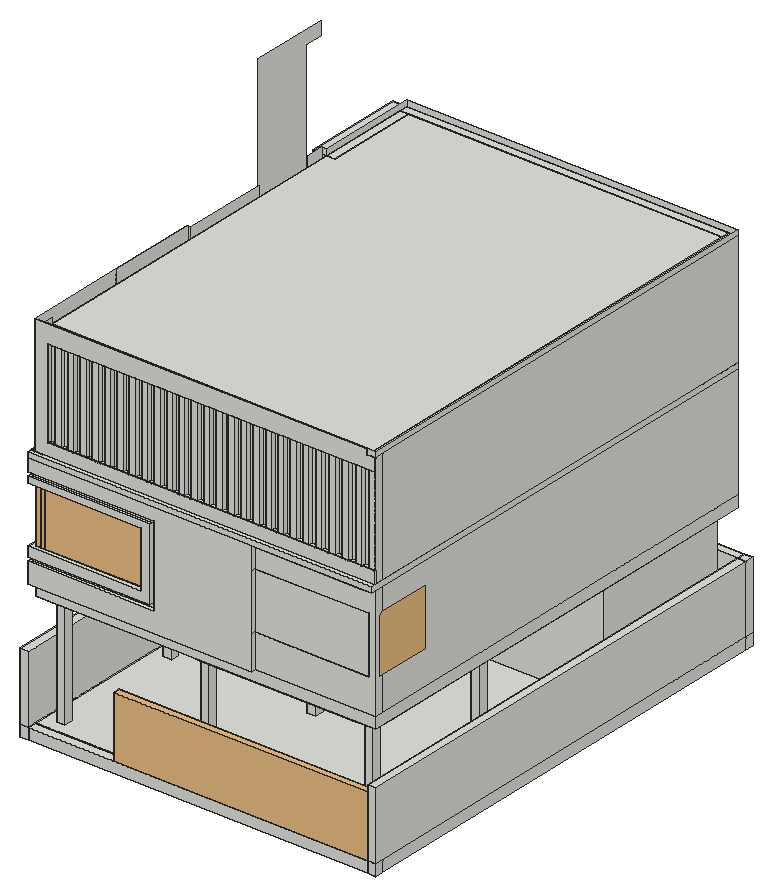
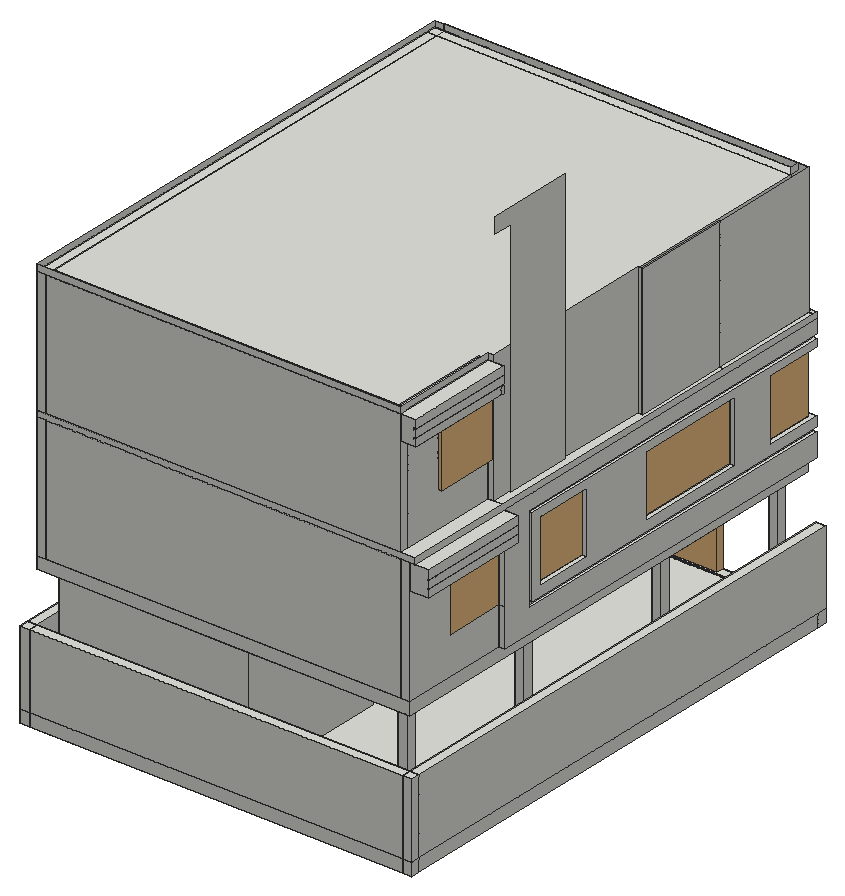
# SketchUp Ruby script. Lengths in inches.
U = 1.inch
M = Sketchup.active_model
def pt(a) = Geom::Point3d.new(a.map { |v| v * U })
def face(e, loops, mat)
  f = e.add_face(loops[0].map { |a| pt(a) })
  loops[1..].each { |l| e.add_face(l.map { |a| pt(a) }).erase! }
  f.material = f.back_material = mat if mat
  f
end
# faces: each face lists its corners as indices into pts; further lists are holes
def faces(e, pts, list, mat = nil) = list.each { |f| face(e, (f[0].is_a?(Array) ? f : [f]).map { |l| l.map { |i| pts[i] } }, mat) }
# xy, xz, yz: faces in a plane at the given z, y or x. An outline is a flat list of corners, or four numbers for a rectangle; further outlines are holes
def ring(l) = l.size == 4 ? [[l[0], l[1]], [l[2], l[1]], [l[2], l[3]], [l[0], l[3]]] : l.each_slice(2).to_a
def flat(e, list, mat, &to3) = list.each { |f| face(e, (f[0].is_a?(Array) ? f : [f]).map { |l| ring(l).map { |u, v| to3.(u, v) } }, mat) }
def xy(e, z, list, mat = nil) = flat(e, list, mat) { |x, y| [x, y, z] }
def xz(e, y, list, mat = nil) = flat(e, list, mat) { |x, z| [x, y, z] }
def yz(e, x, list, mat = nil) = flat(e, list, mat) { |y, z| [x, y, z] }
def lines(e, pts, list) = list.each { |a, b| e.add_line(pt(pts[a]), pt(pts[b])) }
# prism: a flat outline (further loops are holes) pulled along v
def prism(e, loops, v, mat = nil)
  f = face(e, loops, mat); d = Geom::Vector3d.new(v.map { |x| x * U })
  f.pushpull(f.normal.samedirection?(d) ? d.length : -d.length)
end
def box(e, o, s, mat = nil) = prism(e, [[o, [o[0] + s[0], o[1], o[2]], [o[0] + s[0], o[1] + s[1], o[2]], [o[0], o[1] + s[1], o[2]]]], [0, 0, s[2]], mat)
def at(x, y, z, deg = 0) = Geom::Transformation.translation(pt([x, y, z])) * Geom::Transformation.rotation(ORIGIN, Z_AXIS, deg.degrees)
def axes(o, x, y, z) = Geom::Transformation.new([*x, 0, *y, 0, *z, 0, *pt(o).to_a, 1])
def part(name) = M.definitions.add(name)
# library, detail: a bought-in or finely detailed component or shape, given as its bounding box
def library(name, o, s) = part(name).tap { |d| box(d.entities, o, s) }
def detail(e, o, s) = box(e.add_group.entities, o, s)
def put(e, d, t, mat = nil) = e.add_instance(d, t).tap { |i| i.material = mat if mat }
def group(e, t, mat = nil) = e.add_group.tap { |g| g.transformation = t; g.material = mat if mat }.entities
root = M.entities
c1 = library("Garage Gate 243 101",[-254.27,-3.625,0],[508.54,7.25,122.76])
c2 = library("Curtains 004",[-15.59,-2.26,0],[31.18,4.52,116.91])
c3 = library("Window 46-28",[-38.78,-4.09,0],[77.56,5.19,44.09])
c4 = library("Window 46-08",[-34.875,-3.16,0],[69.74,4.26,70.87])
c5 = library("Window 46-05",[-17.86,-2.78,0],[35.72,4.26,58.96])
xy(root,-12,[[9.25,0,18.25,9],[18.25,0,378.25,9],[378.25,0,387.25,9],[9.25,9,18.25,490.375],[18.25,9,378.25,490.375],
  [378.25,9,387.25,490.375],[9.25,490.375,18.25,499.375],[18.25,490.375,378.25,499.375],[378.25,490.375,387.25,499.375]])
xy(root,0,[[9.25,0,18.25,9],[18.25,0,378.25,9],[378.25,0,387.25,9],[9.25,9,18.25,490.375],[18.25,9,378.25,10.375],
  [378.25,9,387.25,490.375],[[18.25,10.375,378.25,490.375],[183.25,328.375,366.25,478.375],[30.25,22.375,39.25,31.375],[183.25,22.375,192.25,31.375],[357.25,22.375,366.25,31.375],[30.25,163.375,39.25,172.375],[183.25,163.375,192.25,172.375],[357.25,163.375,366.25,172.375],[30.25,328.375,39.25,337.375],[30.25,469.375,39.25,478.375]],[30.25,22.375,39.25,31.375],[183.25,22.375,192.25,31.375],[357.25,22.375,366.25,31.375],
  [30.25,163.375,39.25,172.375],[183.25,163.375,192.25,172.375],[357.25,163.375,366.25,172.375],[30.25,328.375,39.25,337.375],[[183.25,328.375,366.25,478.375],[192.25,337.375,357.25,469.375]],
  [192.25,337.375,357.25,469.375],[30.25,469.375,39.25,478.375],[9.25,490.375,18.25,499.375],[18.25,490.375,378.25,499.375],[378.25,490.375,387.25,499.375]])
xy(root,72,[[9.25,0,18.25,490.375],[378.25,0,387.25,490.375],[9.25,490.375,18.25,499.375],[18.25,490.375,378.25,499.375],[378.25,490.375,387.25,499.375]])
xy(root,120,[[18.25,10.375,30.25,31.375],[30.25,10.375,39.25,22.375],[39.25,10.375,183.25,490.375],[183.25,10.375,192.25,22.375],[192.25,10.375,192.25,31.375,183.25,31.375,183.25,163.375,192.25,163.375,192.25,172.375,183.25,172.375,183.25,328.375,378.25,328.375,378.25,172.375,357.25,172.375,357.25,163.375,378.25,163.375,378.25,31.375,357.25,31.375,357.25,10.375],
  [357.25,10.375,378.25,22.375],[30.25,22.375,39.25,31.375],[183.25,22.375,192.25,31.375],[357.25,22.375,366.25,31.375],[366.25,22.375,378.25,31.375],
  [18.25,31.375,39.25,163.375],[18.25,163.375,30.25,172.375],[30.25,163.375,39.25,172.375],[183.25,163.375,192.25,172.375],[357.25,163.375,366.25,172.375],
  [366.25,163.375,378.25,172.375],[18.25,172.375,39.25,328.375],[18.25,328.375,30.25,337.375],[30.25,328.375,39.25,337.375],[[183.25,328.375,366.25,478.375],[192.25,337.375,357.25,469.375]],
  [366.25,328.375,378.25,490.375],[18.25,337.375,39.25,469.375],[18.25,469.375,30.25,490.375],[30.25,469.375,39.25,478.375],[30.25,478.375,39.25,490.375],
  [183.25,478.375,366.25,490.375]])
xy(root,132,[[13.1875,5.3125,18.25,10.375],[18.25,5.3125,27.25,10.375],[27.25,5.3125,250.625,10.375],[13.1875,10.375,18.25,382.375],[18.25,10.375,27.25,490.375],
  [27.25,10.375,378.25,19.375],[27.25,19.375,369.25,481.375],[369.25,19.375,378.25,490.375],[27.25,481.375,369.25,490.375]])
xy(root,154.1875,[[13.1875,5.3125,16.4375,353.0625],[16.4375,5.3125,147.3125,8.5625]])
xy(root,158.1875,[[13.1875,5.3125,16.4375,349.0625],[16.4375,5.3125,143.3125,8.5625]])
xy(root,168,[[13.1875,5.3125,133.375,5.3125,133.375,10.375,18.25,10.375,18.25,62.4375,13.1875,62.4375],[18.25,10.375,27.25,62.4375],[27.25,10.375,133.375,19.375],[250.625,10.375,371.5625,19.375],[369.25,19.375,378.25,75.6875],
  [13.1875,104,18.25,212.1875],[18.25,104,27.25,212.1875],[13.1875,283.375,18.25,340.1875],[18.25,283.375,27.25,340.1875],[18.25,382.375,27.25,442.375]])
xy(root,228,[[13.1875,5.3125,18.25,10.375],[18.25,5.3125,27.25,10.375],[27.25,5.3125,133.375,10.375],[13.1875,10.375,18.25,62.4375],[18.25,10.375,27.25,62.4375],
  [27.25,10.375,133.375,19.375],[250.625,10.375,371.5625,19.375],[369.25,19.375,378.25,75.6875],[13.1875,104,18.25,212.1875],[18.25,104,27.25,212.1875],
  [13.1875,283.375,18.25,340.1875],[18.25,283.375,27.25,340.1875],[0,382.375,0,490.375,18.25,490.375,18.25,487.8125,1.3125,487.8125,1.3125,384.9375,18.25,384.9375,18.25,382.375],[18.25,382.375,27.25,442.375]])
xy(root,229.125,[[1.3125,384.9375,18.25,487.8125]])
xy(root,234.875,[[13.1875,5.3125,16.4375,349.0625],[16.4375,5.3125,143.3125,8.5625]])
xy(root,235.26,[[0,382.375,13.1875,384.375],[0,384.375,1.25,490.375]])
xy(root,236,[[0,382.375,13.1875,384.375],[0,384.375,1.25,490.375]])
xy(root,238.875,[[13.1875,5.3125,16.4375,353.0625]])
xy(root,238.93,[[16.4375,5.3125,147.3125,8.5625]])
xy(root,243.26,[[0,382.375,13.1875,384.375],[0,384.375,1.25,490.375]])
xy(root,244,[[0,382.375,13.1875,384.375],[0,384.375,1.25,490.375]])
xy(root,252,[[13.1875,5.3125,18.25,382.375],[18.25,5.3125,27.25,10.375],[27.25,5.3125,250.625,10.375],[250.625,5.3125,369.25,10.375],[369.25,5.3125,378.25,10.375],
  [18.25,10.375,27.25,490.375],[27.25,10.375,369.25,19.375],[369.25,10.375,378.25,19.375],[27.25,19.375,369.25,481.375],[369.25,19.375,378.25,490.375],
  [0,382.375,13.1875,490.375],[13.1875,382.375,18.25,490.375],[27.25,481.375,369.25,490.375]])
xy(root,258,[[13.1875,5.3125,18.25,9.6875],[18.25,5.3125,27.25,9.6875],[27.25,5.3125,378.25,9.6875],[13.1875,9.6875,17.3125,10.375],[17.3125,9.6875,18.25,10.375],
  [18.25,9.6875,27.25,10.375],[27.25,9.6875,378.25,10.375],[13.1875,10.375,17.3125,117.47],[17.3125,10.375,18.25,117.47],[18.25,10.375,18.25,210.85,22.125,210.85,22.125,300.74,20.6875,300.74,20.6875,365.41,22.125,365.41,22.125,384.4375,27.25,384.4375,27.25,10.375],
  [27.25,10.375,378.25,19.375],[27.25,19.375,369.25,19.375,369.25,481.375,36.25,481.375,36.25,384.4375,27.25,384.4375],[369.25,19.375,378.25,490.375],[13.1875,117.47,17.3125,117.47,17.3125,210.85,22.125,210.85,22.125,300.74,20.6875,300.74,20.6875,365.41,22.125,365.41,22.125,384.4375,13.1875,384.4375],[17.3125,117.47,18.25,210.85],
  [13.1875,384.4375,27.25,490.375],[27.25,384.4375,36.25,481.375],[27.25,481.375,369.25,490.375]])
xy(root,270.81,[[31.06,9.6875,38.27,10.375],[38.27,9.6875,45.19,10.375],[45.19,9.6875,51.4,10.375],[51.4,9.6875,58.32,10.375],[58.32,9.6875,64.52,10.375],
  [64.52,9.6875,71.44,10.375],[71.44,9.6875,77.65,10.375],[77.65,9.6875,84.57,10.375],[84.57,9.6875,90.77,10.375],[90.77,9.6875,97.69,10.375],
  [97.69,9.6875,103.9,10.375],[103.9,9.6875,110.82,10.375],[110.82,9.6875,117.02,10.375],[117.02,9.6875,123.94,10.375],[123.94,9.6875,130.15,10.375],
  [130.15,9.6875,137.07,10.375],[137.07,9.6875,143.27,10.375],[143.27,9.6875,150.19,10.375],[150.19,9.6875,156.4,10.375],[156.4,9.6875,163.32,10.375],
  [163.32,9.6875,169.52,10.375],[169.52,9.6875,176.44,10.375],[176.44,9.6875,182.65,10.375],[182.65,9.6875,189.57,10.375],[189.57,9.6875,195.77,10.375],
  [195.77,9.6875,202.69,10.375],[202.69,9.6875,208.9,10.375],[208.9,9.6875,215.82,10.375],[215.82,9.6875,222.02,10.375],[222.02,9.6875,228.94,10.375],
  [228.94,9.6875,235.15,10.375],[235.15,9.6875,242.07,10.375],[242.07,9.6875,248.27,10.375],[248.27,9.6875,255.19,10.375],[255.19,9.6875,261.4,10.375],
  [261.4,9.6875,268.32,10.375],[268.32,9.6875,274.52,10.375],[274.52,9.6875,281.44,10.375],[281.44,9.6875,287.65,10.375],[287.65,9.6875,294.57,10.375],
  [294.57,9.6875,300.77,10.375],[300.77,9.6875,307.69,10.375],[307.69,9.6875,314.83,10.375],[314.83,9.6875,321.75,10.375],[321.75,9.6875,328.9,10.375],
  [328.9,9.6875,335.82,10.375],[335.82,9.6875,342.96,10.375],[342.96,9.6875,349.88,10.375],[349.88,9.6875,357.02,10.375],[357.02,9.6875,363.94,10.375],
  [363.94,9.6875,371.08,10.375],[371.08,9.6875,378,10.375],[378,9.6875,378.25,10.375],[31.06,10.375,38.27,13.875],[45.19,10.375,51.4,13.875],
  [58.32,10.375,64.52,13.875],[71.44,10.375,77.65,13.875],[84.57,10.375,90.77,13.875],[97.69,10.375,103.9,13.875],[110.82,10.375,117.02,13.875],
  [123.94,10.375,130.15,14.3125],[137.07,10.375,143.27,14.3125],[150.19,10.375,156.4,14.3125],[163.32,10.375,169.52,14.3125],[176.44,10.375,182.65,14.3125],
  [189.57,10.375,195.77,14.3125],[202.69,10.375,208.9,14.3125],[215.82,10.375,222.02,14.3125],[228.94,10.375,235.15,14.3125],[242.07,10.375,248.27,14.3125],
  [255.19,10.375,261.4,14.3125],[268.32,10.375,274.52,14.3125],[281.44,10.375,287.65,14.3125],[294.57,10.375,300.77,14.3125],[307.69,10.375,314.83,14.3125],
  [321.75,10.375,328.9,14.3125],[335.82,10.375,342.96,14.3125],[349.88,10.375,357.02,14.3125],[363.94,10.375,371.08,14.3125]])
xy(root,293.0625,[[27.25,384.4375,36.25,445.375]])
xy(root,354,[[12.6875,384.4375,27.25,387.01],[27.25,384.4375,36.25,445.375],[12.6875,387.01,18.25,487.81],[12.6875,487.81,27.25,490.375]])
xy(root,356.6875,[[18.25,387.01,27.25,487.81]])
xy(root,360.875,[[12.6875,384.4375,18.25,386.4375],[18.25,384.4375,22.125,386.4375],[12.6875,386.4375,13.9375,387.01],[12.6875,387.01,13.9375,490.375]])
xy(root,362,[[12.6875,384.4375,18.25,386.4375],[18.25,384.4375,22.125,386.4375],[12.6875,386.4375,13.9375,490.375]])
xy(root,365.19,[[31.06,9.6875,38.27,10.375],[38.27,9.6875,45.19,10.375],[45.19,9.6875,51.4,10.375],[51.4,9.6875,58.32,10.375],[58.32,9.6875,64.52,10.375],
  [64.52,9.6875,71.44,10.375],[71.44,9.6875,77.65,10.375],[77.65,9.6875,84.57,10.375],[84.57,9.6875,90.77,10.375],[90.77,9.6875,97.69,10.375],
  [97.69,9.6875,103.9,10.375],[103.9,9.6875,110.82,10.375],[110.82,9.6875,117.02,10.375],[117.02,9.6875,123.94,10.375],[123.94,9.6875,130.15,10.375],
  [130.15,9.6875,137.07,10.375],[137.07,9.6875,143.27,10.375],[143.27,9.6875,150.19,10.375],[150.19,9.6875,156.4,10.375],[156.4,9.6875,163.32,10.375],
  [163.32,9.6875,169.52,10.375],[169.52,9.6875,176.44,10.375],[176.44,9.6875,182.65,10.375],[182.65,9.6875,189.57,10.375],[189.57,9.6875,195.77,10.375],
  [195.77,9.6875,202.69,10.375],[202.69,9.6875,208.9,10.375],[208.9,9.6875,215.82,10.375],[215.82,9.6875,222.02,10.375],[222.02,9.6875,228.94,10.375],
  [228.94,9.6875,235.15,10.375],[235.15,9.6875,242.07,10.375],[242.07,9.6875,248.27,10.375],[248.27,9.6875,255.19,10.375],[255.19,9.6875,261.4,10.375],
  [261.4,9.6875,268.32,10.375],[268.32,9.6875,274.52,10.375],[274.52,9.6875,281.44,10.375],[281.44,9.6875,287.65,10.375],[287.65,9.6875,294.57,10.375],
  [294.57,9.6875,300.77,10.375],[300.77,9.6875,307.69,10.375],[307.69,9.6875,314.83,10.375],[314.83,9.6875,321.75,10.375],[321.75,9.6875,328.9,10.375],
  [328.9,9.6875,335.82,10.375],[335.82,9.6875,342.96,10.375],[342.96,9.6875,349.88,10.375],[349.88,9.6875,357.02,10.375],[357.02,9.6875,363.94,10.375],
  [363.94,9.6875,371.08,10.375],[371.08,9.6875,378,10.375],[378,9.6875,378.25,10.375],[31.06,10.375,38.27,13.875],[45.19,10.375,51.4,13.875],
  [58.32,10.375,64.52,13.875],[71.44,10.375,77.65,13.875],[84.57,10.375,90.77,13.875],[97.69,10.375,103.9,13.875],[110.82,10.375,117.02,13.875],
  [123.94,10.375,130.15,14.3125],[137.07,10.375,143.27,14.3125],[150.19,10.375,156.4,14.3125],[163.32,10.375,169.52,14.3125],[176.44,10.375,182.65,14.3125],
  [189.57,10.375,195.77,14.3125],[202.69,10.375,208.9,14.3125],[215.82,10.375,222.02,14.3125],[228.94,10.375,235.15,14.3125],[242.07,10.375,248.27,14.3125],
  [255.19,10.375,261.4,14.3125],[268.32,10.375,274.52,14.3125],[281.44,10.375,287.65,14.3125],[294.57,10.375,300.77,14.3125],[307.69,10.375,314.83,14.3125],
  [321.75,10.375,328.9,14.3125],[335.82,10.375,342.96,14.3125],[349.88,10.375,357.02,14.3125],[363.94,10.375,371.08,14.3125]])
xy(root,368.875,[[12.6875,384.4375,18.25,386.4375],[18.25,384.4375,22.125,386.4375],[12.6875,386.4375,13.9375,490.375]])
xy(root,370,[[12.6875,384.4375,18.25,386.4375],[18.25,384.4375,22.125,386.4375],[12.6875,386.4375,13.9375,490.375]])
xy(root,378,[[369.25,9.6875,378.25,10.375],[27.25,10.375,369.25,19.375],[369.25,10.375,378.25,19.375],[27.25,19.375,27.25,384.4375,36.25,384.4375,36.25,481.375,369.25,481.375,369.25,19.375],[369.25,19.375,378.25,490.375],
  [12.6875,384.4375,27.25,490.375],[27.25,384.4375,36.25,481.375],[27.25,481.375,369.25,490.375]])
xz(root,0,[[9.25,-12,18.25,0],[18.25,-12,378.25,0],[378.25,-12,387.25,0],[9.25,0,18.25,72],[378.25,0,387.25,72]])
xz(root,5.3125,[[13.1875,132,250.625,132,250.625,252,13.1875,252,13.1875,238.875,16.4375,238.875,16.4375,238.93,147.3125,238.93,147.3125,154.1875,13.1875,154.1875],[13.1875,158.1875,143.3125,158.1875,143.3125,234.875,13.1875,234.875,13.1875,228,133.375,228,133.375,168,13.1875,168],[13.1875,252,378.25,258]])
xz(root,8.5625,[[16.4375,154.1875,147.3125,154.1875,147.3125,238.93,16.4375,238.93,16.4375,234.875,143.3125,234.875,143.3125,158.1875,16.4375,158.1875]])
xz(root,9,[[9.25,-12,18.25,0],[18.25,-12,378.25,0],[378.25,-12,387.25,0]])
xz(root,9.6875,[[17.3125,258,378.25,258,378.25,270.81,31.06,270.81,31.06,365.19,378.25,365.19,378.25,378,369.25,378,369.25,383.75,17.3125,383.75]])
xz(root,10.375,[[18.25,120,378.25,132],[18.25,132,18.25,168,133.375,168,133.375,228,18.25,228,18.25,252,250.625,252,250.625,132],[250.625,132,378.25,132,378.25,252,250.625,252,250.625,228,371.5625,228,371.5625,168,250.625,168],[250.625,168,371.5625,228],[18.25,258,18.25,384,27.25,384,27.25,378,378.25,378,378.25,365.19,31.06,365.19,31.06,270.81,378.25,270.81,378.25,258],
  [38.27,270.81,45.19,365.19],[51.4,270.81,58.32,365.19],[64.52,270.81,71.44,365.19],[77.65,270.81,84.57,365.19],[90.77,270.81,97.69,365.19],
  [103.9,270.81,110.82,365.19],[117.02,270.81,123.94,365.19],[130.15,270.81,137.07,365.19],[143.27,270.81,150.19,365.19],[156.4,270.81,163.32,365.19],
  [169.52,270.81,176.44,365.19],[182.65,270.81,189.57,365.19],[195.77,270.81,202.69,365.19],[208.9,270.81,215.82,365.19],[222.02,270.81,228.94,365.19],
  [235.15,270.81,242.07,365.19],[248.27,270.81,255.19,365.19],[261.4,270.81,268.32,365.19],[274.52,270.81,281.44,365.19],[287.65,270.81,294.57,365.19],
  [300.77,270.81,307.69,365.19],[314.83,270.81,321.75,365.19],[328.9,270.81,335.82,365.19],[342.96,270.81,349.88,365.19],[357.02,270.81,363.94,365.19],
  [371.08,270.81,378,365.19],[378,270.81,378.25,365.19],[27.25,378,369.25,384],[369.25,378,378.25,384]])
xz(root,13.875,[[31.06,270.81,38.27,365.19],[45.19,270.81,51.4,365.19],[58.32,270.81,64.52,365.19],[71.44,270.81,77.65,365.19],[84.57,270.81,90.77,365.19],
  [97.69,270.81,103.9,365.19],[110.82,270.81,117.02,365.19]])
xz(root,14.3125,[[123.94,270.81,130.15,365.19],[137.07,270.81,143.27,365.19],[150.19,270.81,156.4,365.19],[163.32,270.81,169.52,365.19],[176.44,270.81,182.65,365.19],
  [189.57,270.81,195.77,365.19],[202.69,270.81,208.9,365.19],[215.82,270.81,222.02,365.19],[228.94,270.81,235.15,365.19],[242.07,270.81,248.27,365.19],
  [255.19,270.81,261.4,365.19],[268.32,270.81,274.52,365.19],[281.44,270.81,287.65,365.19],[294.57,270.81,300.77,365.19],[307.69,270.81,314.83,365.19],
  [321.75,270.81,328.9,365.19],[335.82,270.81,342.96,365.19],[349.88,270.81,357.02,365.19],[363.94,270.81,371.08,365.19]])
xz(root,19.375,[[27.25,132,27.25,168,133.375,168,133.375,228,27.25,228,27.25,252,369.25,252,369.25,228,250.625,228,250.625,168,369.25,168,369.25,132],[369.25,132,378.25,168],[369.25,168,371.5625,228],[371.5625,168,378.25,228],[369.25,228,378.25,252],
  [27.25,258,369.25,378],[369.25,258,378.25,378]])
xz(root,22.375,[[30.25,0,39.25,120],[183.25,0,192.25,120],[357.25,0,366.25,120]])
xz(root,31.375,[[30.25,0,39.25,120],[183.25,0,192.25,120],[357.25,0,366.25,120]])
xz(root,62.4375,[[13.1875,168,18.25,228],[18.25,168,27.25,228]])
xz(root,75.6875,[[369.25,168,378.25,228]])
xz(root,104,[[13.1875,168,18.25,228],[18.25,168,27.25,228]])
xz(root,117.47,[[17.3125,258,18.25,384]])
xz(root,163.375,[[30.25,0,39.25,120],[183.25,0,192.25,120],[357.25,0,366.25,120]])
xz(root,172.375,[[30.25,0,39.25,120],[183.25,0,192.25,120],[357.25,0,366.25,120]])
xz(root,210.85,[[17.3125,258,18.25,384],[18.25,258,22.125,384]])
xz(root,212.1875,[[13.1875,168,18.25,228],[18.25,168,27.25,228]])
xz(root,283.375,[[13.1875,168,18.25,228],[18.25,168,27.25,228]])
xz(root,300.74,[[20.6875,258,22.125,384]])
xz(root,328.375,[[30.25,0,39.25,120],[183.25,0,366.25,120]])
xz(root,337.375,[[30.25,0,39.25,120],[192.25,0,357.25,120]])
xz(root,340.1875,[[13.1875,168,18.25,228],[18.25,168,27.25,228]])
xz(root,349.0625,[[13.1875,158.1875,16.4375,234.875]])
xz(root,353.0625,[[13.1875,154.1875,16.4375,238.875]])
xz(root,365.41,[[20.6875,258,22.125,384]])
xz(root,382.375,[[13.1875,132,18.25,168],[13.1875,168,18.25,228],[18.25,168,27.25,228],[0,228,13.1875,235.26],[13.1875,228,18.25,252],
  [0,236,13.1875,243.26],[0,244,13.1875,252]])
xz(root,384.375,[[1.25,235.26,13.1875,236],[1.25,243.26,13.1875,244]])
xz(root,384.4375,[[22.125,258,27.25,354],[27.25,258,36.25,293.0625],[27.25,293.0625,36.25,354],[12.6875,354,22.125,360.875],[22.125,354,27.25,378],
  [27.25,354,36.25,378],[12.6875,362,22.125,368.875],[12.6875,370,22.125,378],[22.125,378,27.25,384]])
xz(root,384.9375,[[1.3125,228,13.1875,229.125],[13.1875,228,18.25,229.125]])
xz(root,386.4375,[[13.9375,360.875,18.25,362],[18.25,360.875,22.125,362],[13.9375,368.875,18.25,370],[18.25,368.875,22.125,370]])
xz(root,387.01,[[18.25,354,27.25,356.6875]])
xz(root,442.375,[[18.25,168,27.25,228]])
xz(root,445.375,[[27.25,293.0625,36.25,354]])
xz(root,469.375,[[30.25,0,39.25,120],[192.25,0,357.25,120]])
xz(root,478.375,[[30.25,0,39.25,120],[183.25,0,366.25,120]])
xz(root,481.375,[[27.25,132,369.25,252],[27.25,258,36.25,378],[36.25,258,369.25,378]])
xz(root,487.81,[[18.25,354,27.25,356.6875]])
xz(root,487.8125,[[1.3125,228,18.25,229.125]])
xz(root,490.375,[[9.25,-12,18.25,0],[18.25,-12,378.25,0],[378.25,-12,387.25,0],[9.25,0,18.25,72],[18.25,0,378.25,72],
  [378.25,0,387.25,72],[18.25,120,378.25,132],[18.25,132,27.25,252],[27.25,132,369.25,252],[369.25,132,378.25,252],
  [0,228,0,235.26,1.25,235.26,1.25,236,0,236,0,243.26,1.25,243.26,1.25,244,0,244,0,252,18.25,252,18.25,228],[13.1875,252,378.25,258],[27.25,258,369.25,378],[369.25,258,378.25,378],[12.6875,354,12.6875,360.875,13.9375,360.875,13.9375,362,12.6875,362,12.6875,368.875,13.9375,368.875,13.9375,370,12.6875,370,12.6875,378,27.25,378,27.25,354],
  [27.25,378,378.25,384]])
xz(root,499.375,[[9.25,-12,18.25,0],[18.25,-12,378.25,0],[378.25,-12,387.25,0],[9.25,0,18.25,72],[18.25,0,378.25,72],
  [378.25,0,387.25,72]])
yz(root,0,[[382.375,228,490.375,235.26],[382.375,236,490.375,243.26],[382.375,244,490.375,252]])
yz(root,1.25,[[384.375,235.26,490.375,236],[384.375,243.26,490.375,244]])
yz(root,1.3125,[[384.9375,228,487.8125,229.125]])
yz(root,9.25,[[0,-12,9,0],[9,-12,490.375,0],[490.375,-12,499.375,0],[0,0,490.375,72],[490.375,0,499.375,72]])
yz(root,12.6875,[[384.4375,354,387.01,360.875],[387.01,354,490.375,360.875],[384.4375,362,490.375,368.875],[384.4375,370,490.375,378]])
yz(root,13.1875,[[5.3125,132,5.3125,154.1875,353.0625,154.1875,353.0625,238.875,5.3125,238.875,5.3125,252,382.375,252,382.375,132],[[5.3125,158.1875,5.3125,168,62.4375,168,62.4375,228,5.3125,228,5.3125,234.875,349.0625,234.875,349.0625,158.1875],[104,168,212.1875,228],[283.375,168,340.1875,228]],[382.375,235.26,384.375,236],[382.375,243.26,384.375,244],[5.3125,252,490.375,258]])
yz(root,13.9375,[[386.4375,360.875,490.375,362],[386.4375,368.875,490.375,370]])
yz(root,16.4375,[[8.5625,154.1875,8.5625,158.1875,349.0625,158.1875,349.0625,234.875,8.5625,234.875,8.5625,238.875,353.0625,238.875,353.0625,154.1875],[5.3125,238.875,8.5625,238.93]])
yz(root,17.3125,[[9.6875,258,117.47,383.75],[117.47,258,210.85,383.75]])
yz(root,18.25,[[0,-12,9,0],[9,-12,490.375,0],[490.375,-12,499.375,0],[0,0,490.375,72],[490.375,0,499.375,72],
  [10.375,120,490.375,132],[[10.375,132,382.375,132,382.375,252,10.375,252,10.375,228,62.4375,228,62.4375,168,10.375,168],[104,168,212.1875,228],[283.375,168,340.1875,228]],[382.375,132,382.375,168,442.375,168,442.375,229.125,487.8125,229.125,487.8125,228,490.375,228,490.375,132],[382.375,228,384.9375,228,384.9375,229.125,487.8125,229.125,487.8125,228,490.375,228,490.375,252,382.375,252],[384.9375,228,442.375,229.125],
  [117.47,258,210.85,384],[387.01,354,487.81,356.6875]])
yz(root,20.6875,[[300.74,258,300.74,504,384.4375,504,384.4375,488.88,365.41,488.88,365.41,258]])
yz(root,22.125,[[210.85,258,300.74,384],[365.41,258,384.4375,384],[384.4375,360.875,386.4375,362],[384.4375,368.875,386.4375,370]])
yz(root,27.25,[[[19.375,132,481.375,132,481.375,252,19.375,252,19.375,228,62.4375,228,62.4375,168,19.375,168],[104,168,212.1875,228],[382.375,168,442.375,228],[283.375,168,340.1875,228]],[481.375,132,490.375,252],[19.375,258,384.4375,378],[384.4375,258,384.4375,293.0625,445.375,293.0625,445.375,356.6875,481.375,356.6875,481.375,258],[481.375,258,481.375,356.6875,487.81,356.6875,487.81,354,490.375,354,490.375,258],
  [384.4375,354,387.01,354,387.01,356.6875,481.375,356.6875,481.375,378,384.4375,378],[387.01,354,445.375,356.6875],[487.81,354,487.81,356.6875,481.375,356.6875,481.375,378,490.375,378,490.375,354],[10.375,378,19.375,384],[384.4375,378,490.375,384]])
yz(root,30.25,[[22.375,0,31.375,120],[163.375,0,172.375,120],[328.375,0,337.375,120],[469.375,0,478.375,120]])
yz(root,31.06,[[9.6875,270.81,10.375,365.19],[10.375,270.81,13.875,365.19]])
yz(root,36.25,[[384.4375,258,481.375,258,481.375,378,384.4375,378,384.4375,354,445.375,354,445.375,293.0625,384.4375,293.0625]])
yz(root,38.27,[[10.375,270.81,13.875,365.19]])
yz(root,39.25,[[22.375,0,31.375,120],[163.375,0,172.375,120],[328.375,0,337.375,120],[469.375,0,478.375,120]])
yz(root,45.19,[[10.375,270.81,13.875,365.19]])
yz(root,51.4,[[10.375,270.81,13.875,365.19]])
yz(root,58.32,[[10.375,270.81,13.875,365.19]])
yz(root,64.52,[[10.375,270.81,13.875,365.19]])
yz(root,71.44,[[10.375,270.81,13.875,365.19]])
yz(root,77.65,[[10.375,270.81,13.875,365.19]])
yz(root,84.57,[[10.375,270.81,13.875,365.19]])
yz(root,90.77,[[10.375,270.81,13.875,365.19]])
yz(root,97.69,[[10.375,270.81,13.875,365.19]])
yz(root,103.9,[[10.375,270.81,13.875,365.19]])
yz(root,110.82,[[10.375,270.81,13.875,365.19]])
yz(root,117.02,[[10.375,270.81,13.875,365.19]])
yz(root,123.94,[[10.375,270.81,14.3125,365.19]])
yz(root,130.15,[[10.375,270.81,14.3125,365.19]])
yz(root,133.375,[[5.3125,168,10.375,228],[10.375,168,19.375,228]])
yz(root,137.07,[[10.375,270.81,14.3125,365.19]])
yz(root,143.27,[[10.375,270.81,14.3125,365.19]])
yz(root,143.3125,[[5.3125,158.1875,8.5625,234.875]])
yz(root,147.3125,[[5.3125,154.1875,8.5625,238.93]])
yz(root,150.19,[[10.375,270.81,14.3125,365.19]])
yz(root,156.4,[[10.375,270.81,14.3125,365.19]])
yz(root,163.32,[[10.375,270.81,14.3125,365.19]])
yz(root,169.52,[[10.375,270.81,14.3125,365.19]])
yz(root,176.44,[[10.375,270.81,14.3125,365.19]])
yz(root,182.65,[[10.375,270.81,14.3125,365.19]])
yz(root,183.25,[[22.375,0,31.375,120],[163.375,0,172.375,120],[328.375,0,478.375,120]])
yz(root,189.57,[[10.375,270.81,14.3125,365.19]])
yz(root,192.25,[[22.375,0,31.375,120],[163.375,0,172.375,120],[337.375,0,469.375,120]])
yz(root,195.77,[[10.375,270.81,14.3125,365.19]])
yz(root,202.69,[[10.375,270.81,14.3125,365.19]])
yz(root,208.9,[[10.375,270.81,14.3125,365.19]])
yz(root,215.82,[[10.375,270.81,14.3125,365.19]])
yz(root,222.02,[[10.375,270.81,14.3125,365.19]])
yz(root,228.94,[[10.375,270.81,14.3125,365.19]])
yz(root,235.15,[[10.375,270.81,14.3125,365.19]])
yz(root,242.07,[[10.375,270.81,14.3125,365.19]])
yz(root,248.27,[[10.375,270.81,14.3125,365.19]])
yz(root,250.625,[[5.3125,132,10.375,168],[5.3125,168,10.375,228],[10.375,168,19.375,228],[5.3125,228,10.375,252]])
yz(root,255.19,[[10.375,270.81,14.3125,365.19]])
yz(root,261.4,[[10.375,270.81,14.3125,365.19]])
yz(root,268.32,[[10.375,270.81,14.3125,365.19]])
yz(root,274.52,[[10.375,270.81,14.3125,365.19]])
yz(root,281.44,[[10.375,270.81,14.3125,365.19]])
yz(root,287.65,[[10.375,270.81,14.3125,365.19]])
yz(root,294.57,[[10.375,270.81,14.3125,365.19]])
yz(root,300.77,[[10.375,270.81,14.3125,365.19]])
yz(root,307.69,[[10.375,270.81,14.3125,365.19]])
yz(root,314.83,[[10.375,270.81,14.3125,365.19]])
yz(root,321.75,[[10.375,270.81,14.3125,365.19]])
yz(root,328.9,[[10.375,270.81,14.3125,365.19]])
yz(root,335.82,[[10.375,270.81,14.3125,365.19]])
yz(root,342.96,[[10.375,270.81,14.3125,365.19]])
yz(root,349.88,[[10.375,270.81,14.3125,365.19]])
yz(root,357.02,[[10.375,270.81,14.3125,365.19]])
yz(root,357.25,[[22.375,0,31.375,120],[163.375,0,172.375,120],[337.375,0,469.375,120]])
yz(root,363.94,[[10.375,270.81,14.3125,365.19]])
yz(root,366.25,[[22.375,0,31.375,120],[163.375,0,172.375,120],[328.375,0,478.375,120]])
yz(root,369.25,[[19.375,132,19.375,168,75.6875,168,75.6875,228,19.375,228,19.375,252,481.375,252,481.375,132],[481.375,132,490.375,252],[19.375,258,481.375,378],[481.375,258,490.375,378],[9.6875,378,10.375,384]])
yz(root,371.08,[[10.375,270.81,14.3125,365.19]])
yz(root,371.5625,[[10.375,168,19.375,228]])
yz(root,378.25,[[0,-12,9,0],[9,-12,490.375,0],[490.375,-12,499.375,0],[0,0,490.375,72],[490.375,0,499.375,72],
  [10.375,120,490.375,132],[10.375,132,19.375,252],[19.375,132,490.375,132,490.375,252,19.375,252,19.375,228,75.6875,228,75.6875,168,19.375,168],[5.3125,252,490.375,258],[9.6875,258,10.375,270.81],
  [10.375,258,19.375,378],[19.375,258,490.375,378],[9.6875,365.19,10.375,378],[10.375,378,490.375,384]])
yz(root,387.25,[[0,-12,9,0],[9,-12,490.375,0],[490.375,-12,499.375,0],[0,0,490.375,72],[490.375,0,499.375,72]])
p = [[18.25,10.375,168],[18.25,10.375,228]]
lines(root,p,[[0,1]])
put(root,c1,axes([243.49,3.6,-0.02],[0.53,0,0],[0,1,0],[0,0,0.5292]))
put(root,c2,at(27.45,430.59,130.58,90))
put(root,c2,at(29.51,389.35,135.09,90))
put(root,c2,at(27.44,336.07,135.09,90))
put(root,c2,at(27.44,118.7,135.09,90))
put(root,c2,at(27.44,196.7,135.09,90))
put(root,c2,at(27.44,51.82,135.09,90))
put(root,c2,at(118.66,21.63,135.09))
put(root,c2,at(264.98,21.63,135.09))
put(root,c2,at(296.1,21.63,135.09))
put(root,c2,at(321.79,21.63,135.09))
put(root,c3,axes([19.35,158.09,168],[0,1.39497,0],[-1,0,0],[0,0,1.36088]))
put(root,c4,axes([19.35,412.375,168],[0,0.86027,0],[-1,0,0],[0,0,0.84667]))
put(root,c5,axes([375.16,46.14,168],[0,-1.65366,0],[2.0916,0,0],[0,0,1.02]))
put(root,c5,axes([22.86,311.78,168],[0,-1.59006,0],[1.66,0,0],[0,0,1]))
put(root,c4,axes([78.47,11.48,168],[-1.57438,0,0],[0,-1,0],[0,0,0.84667]))
put(root,c3,axes([311.09,11.48,168],[-1.55937,0,0],[0,-1,0],[0,0,1.36088]))
put(root,c5,axes([24.0625,38.78,168],[0,-1.59006,0],[2.0916,0,0],[0,0,1]))
put(root,c4,axes([24.09,415.375,293.0625],[0,0.86027,0],[-1,0,0],[0,0,0.84667]))
